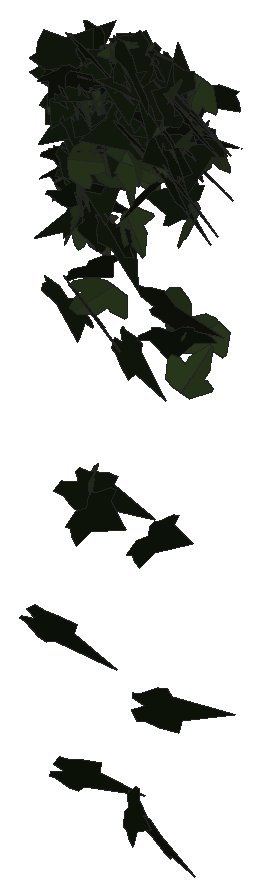
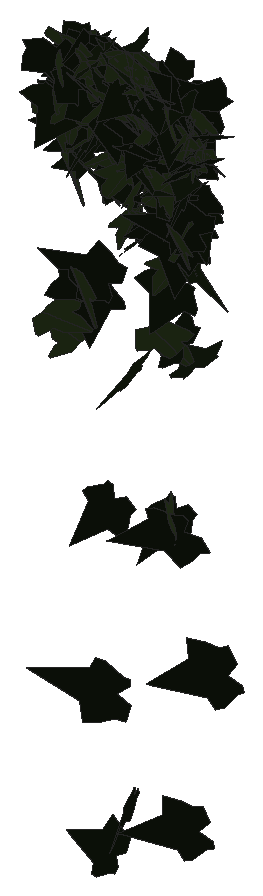
# SketchUp Ruby script. Lengths in inches.
U = 1.inch
M = Sketchup.active_model
def pt(a) = Geom::Point3d.new(a.map { |v| v * U })
def face(e, loops, mat)
  f = e.add_face(loops[0].map { |a| pt(a) })
  loops[1..].each { |l| e.add_face(l.map { |a| pt(a) }).erase! }
  f.material = f.back_material = mat if mat
  f
end
# faces: each face lists its corners as indices into pts; further lists are holes
def faces(e, pts, list, mat = nil) = list.each { |f| face(e, (f[0].is_a?(Array) ? f : [f]).map { |l| l.map { |i| pts[i] } }, mat) }
# xy, xz, yz: faces in a plane at the given z, y or x. An outline is a flat list of corners, or four numbers for a rectangle; further outlines are holes
def ring(l) = l.size == 4 ? [[l[0], l[1]], [l[2], l[1]], [l[2], l[3]], [l[0], l[3]]] : l.each_slice(2).to_a
def flat(e, list, mat, &to3) = list.each { |f| face(e, (f[0].is_a?(Array) ? f : [f]).map { |l| ring(l).map { |u, v| to3.(u, v) } }, mat) }
def xy(e, z, list, mat = nil) = flat(e, list, mat) { |x, y| [x, y, z] }
def xz(e, y, list, mat = nil) = flat(e, list, mat) { |x, z| [x, y, z] }
def yz(e, x, list, mat = nil) = flat(e, list, mat) { |y, z| [x, y, z] }
def lines(e, pts, list) = list.each { |a, b| e.add_line(pt(pts[a]), pt(pts[b])) }
# prism: a flat outline (further loops are holes) pulled along v
def prism(e, loops, v, mat = nil)
  f = face(e, loops, mat); d = Geom::Vector3d.new(v.map { |x| x * U })
  f.pushpull(f.normal.samedirection?(d) ? d.length : -d.length)
end
def box(e, o, s, mat = nil) = prism(e, [[o, [o[0] + s[0], o[1], o[2]], [o[0] + s[0], o[1] + s[1], o[2]], [o[0], o[1] + s[1], o[2]]]], [0, 0, s[2]], mat)
def at(x, y, z, deg = 0) = Geom::Transformation.translation(pt([x, y, z])) * Geom::Transformation.rotation(ORIGIN, Z_AXIS, deg.degrees)
def axes(o, x, y, z) = Geom::Transformation.new([*x, 0, *y, 0, *z, 0, *pt(o).to_a, 1])
def part(name) = M.definitions.add(name)
# library, detail: a bought-in or finely detailed component or shape, given as its bounding box
def library(name, o, s) = part(name).tap { |d| box(d.entities, o, s) }
def detail(e, o, s) = box(e.add_group.entities, o, s)
def put(e, d, t, mat = nil) = e.add_instance(d, t).tap { |i| i.material = mat if mat }
def group(e, t, mat = nil) = e.add_group.tap { |g| g.transformation = t; g.material = mat if mat }.entities
root = M.entities
M.materials.add("1026 AP 7946 SUNNY SIDE UP").color = [254, 231, 186]
M.materials.add("efeu1").color = [18, 25, 13]
M.materials.add("efeu2").color = [43, 57, 29]
c1 = part("ivyleaf_9")
p = [[1.54,2.16,1.25],[1.36,2.04,1.19],[-0.21,0.99,0.68],[-0.71,1.11,0.82],[-0.85,0.86,0.67],[-0.8,0.17,0.21],
  [-0.9,-0.01,0.1],[-0.67,-0.16,-0.02],[-0.08,-0.08,-0.05],[-0.03,-0.6,-0.4],[0.65,-0.88,-0.66],[0.83,-0.6,-0.49],
  [1.29,-0.42,-0.43],[1.8125,-0.07,-0.26],[1.21,0.44,0.15]]
faces(c1.entities,p,[[0,1,2,3,4,5,6,7,8,9,10,11,12,13,14]],"efeu1")
c2 = part("ivyleaf_10")
p = [[0,0.5,-0.03],[-0.0625,2.02,-0.43],[-0.19,2.01,-0.46],[-0.54,1.05,-0.29],[-0.52,0.625,-0.18],[-0.83,0.76,-0.28],
  [-1.16,0.64,-0.33],[-1.15,0.33,-0.24],[-0.77,-0.39,0.02],[-0.3,-0.51,0.16],[0.04,-0.48,0.23],[-0.02,2.01,-0.4375],
  [-0.06,2.01,-0.43],[0.04,-0.49,0.23],[0.67,-0.49,0.14],[1.38,0.36,-0.2],[1.375,0.51,-0.24],[0.81,0.65,-0.19],
  [0.62,0.59,-0.15],[0.6,1.09,-0.28],[0.5,1.23,-0.31]]
faces(c2.entities,p,[[0,1,2,3,4,5,6,7,8,9,10],[11,12,0,13,14,15,16,17,18,19,20]],"efeu2")
put(root,c1,axes([115.99,212.79,265.13],[-0.26427,0.17378,-0.05121],[0.02717,-0.05346,-0.24811],[-0.28334,-0.16721,0.02397]),"1026 AP 7946 SUNNY SIDE UP")
put(root,c1,axes([115.74,212.99,266.61],[-0.0821,-0.23949,0.03265],[-0.00331,-0.03337,-0.25266],[0.38014,-0.05201,0.00485]),"1026 AP 7946 SUNNY SIDE UP")
put(root,c2,axes([115.73,212.88,266.77],[0.19919,0.21849,0.01482],[0.02802,0.00485,-0.25981],[-0.34304,0.12727,-0.01262]),"1026 AP 7946 SUNNY SIDE UP")
put(root,c1,axes([115.8125,212.93,267.01],[-0.23551,-0.2009,0.04173],[0.02399,-0.06233,-0.25357],[0.32172,-0.14242,0.04946]),"1026 AP 7946 SUNNY SIDE UP")
put(root,c1,axes([115.93,212.68,265.9],[0.01878,0.24384,-0.04183],[-0.01659,-0.0415,-0.2516],[-0.38871,0.01355,0.00872]),"1026 AP 7946 SUNNY SIDE UP")
put(root,c2,axes([115.85,212.9,265.35],[0.05116,0.23767,-0.06271],[0.01151,0.0618,0.24749],[0.38613,-0.03333,0.00093]),"1026 AP 7946 SUNNY SIDE UP")
put(root,c1,axes([115.81,212.93,266.33],[0.24825,-0.13578,-0.18185],[-0.24069,0.08971,-0.21253],[0.25302,0.21856,-0.02375]),"1026 AP 7946 SUNNY SIDE UP")
put(root,c1,axes([115.68,212.91,263.6875],[-0.0167,-0.20611,0.14387],[0.09275,-0.13903,-0.20586],[0.38139,0.02479,0.05636]),"1026 AP 7946 SUNNY SIDE UP")
put(root,c1,axes([115.52,212.53,258.98],[0.41358,-0.02859,0.1247],[0.18193,-0.04871,-0.27076],[0.07246,0.28548,-0.03197]),"1026 AP 7946 SUNNY SIDE UP")
put(root,c2,axes([115.88,213.13,265.69],[0.27606,-0.17043,-0.00359],[-0.02245,-0.01111,-0.25146],[0.26707,0.17523,-0.01743]),"1026 AP 7946 SUNNY SIDE UP")
put(root,c2,axes([115.83,212.89,267.06],[-0.03773,0.24961,-0.05464],[0.00008,-0.05469,-0.2586],[-0.40172,-0.02346,0.00508]),"1026 AP 7946 SUNNY SIDE UP")
put(root,c1,axes([115.65,213,266.52],[0.28935,-0.16498,-0.02634],[0.01885,0.04965,-0.25011],[0.26162,0.17889,0.04715]),"1026 AP 7946 SUNNY SIDE UP")
put(root,c2,axes([115.875,212.79,267.35],[0.37173,-0.10682,0.00444],[-0.00745,-0.02238,-0.26639],[0.16798,0.2354,-0.02164]),"1026 AP 7946 SUNNY SIDE UP")
put(root,c2,axes([115.79,212.91,266.5625],[-0.13441,0.1576,-0.18274],[0.10829,-0.16494,-0.18519],[-0.35814,-0.10902,0.01259]),"1026 AP 7946 SUNNY SIDE UP")
put(root,c1,axes([115.74,212.92,266.82],[0.10246,-0.24103,0.0478],[-0.00107,-0.04959,-0.25714],[0.38636,0.06378,-0.01339]),"1026 AP 7946 SUNNY SIDE UP")
put(root,c1,axes([115.64,212.97,265.6875],[0.15087,0.01394,0.23225],[0.35005,0.03508,-0.09967],[-0.05933,0.24241,0.00252]),"1026 AP 7946 SUNNY SIDE UP")
put(root,c2,axes([116.03,212.91,267.03],[0.28883,-0.12781,-0.12018],[-0.14742,0.06823,-0.23013],[0.22779,0.20622,0.00345]),"1026 AP 7946 SUNNY SIDE UP")
put(root,c1,axes([115.96,212.9,265.45],[0.15048,0.22625,-0.03636],[-0.00526,-0.03826,-0.25301],[-0.36034,0.09504,-0.01149]),"1026 AP 7946 SUNNY SIDE UP")
put(root,c1,axes([116.01,212.66,266.07],[0.25903,0.14712,-0.11483],[-0.12722,-0.07798,-0.22796],[-0.26175,0.18349,-0.00284]),"1026 AP 7946 SUNNY SIDE UP")
put(root,c1,axes([115.75,212.83,266.95],[0.19134,-0.21265,0.06418],[0.04405,-0.05713,-0.2527],[0.34617,0.12481,-0.00332]),"1026 AP 7946 SUNNY SIDE UP")
put(root,c1,axes([115.83,212.66,267.36],[-0.1452,-0.01813,0.27512],[0.39855,0.08523,0.09671],[-0.13579,0.26952,-0.01033]),"1026 AP 7946 SUNNY SIDE UP")
put(root,c1,axes([115.84,212.97,266.64],[-0.1131,-0.19479,-0.14542],[0.14339,0.11304,-0.20955],[0.34892,-0.10959,0.03898]),"1026 AP 7946 SUNNY SIDE UP")
put(root,c1,axes([116.11,212.56,267.42],[0.03387,0.22555,-0.15246],[-0.01506,-0.14902,-0.23425],[-0.42503,0.02325,-0.00385]),"1026 AP 7946 SUNNY SIDE UP")
put(root,c2,axes([115.97,212.67,265.74],[-0.22116,0.20193,-0.02831],[0.00589,-0.03221,-0.25322],[-0.32063,-0.13987,0.01488]),"1026 AP 7946 SUNNY SIDE UP")
put(root,c2,axes([116.05,212.9,266.75],[-0.38906,-0.02119,0.00829],[-0.00969,-0.0233,-0.2549],[0.03437,-0.24646,0.02192]),"1026 AP 7946 SUNNY SIDE UP")
put(root,c2,axes([115.85,212.77,267.05],[0.24228,-0.14413,0.1453],[0.20469,-0.0658,-0.21491],[0.24335,0.19884,0.0361]),"1026 AP 7946 SUNNY SIDE UP")
put(root,c1,axes([115.91,212.76,266.07],[0.14209,-0.18673,-0.17045],[-0.12451,0.14422,-0.21275],[0.37084,0.11997,-0.00612]),"1026 AP 7946 SUNNY SIDE UP")
put(root,c1,axes([115.97,212.8,267.56],[0.3184,-0.03652,-0.16831],[-0.21748,0.10742,-0.20096],[0.14774,0.23683,0.0669]),"1026 AP 7946 SUNNY SIDE UP")
put(root,c2,axes([115.91,212.82,267.04],[-0.16774,0.12497,-0.19879],[0.14491,-0.17248,-0.16796],[-0.33219,-0.13834,0.02711]),"1026 AP 7946 SUNNY SIDE UP")
put(root,c1,axes([116.12,212.88,267.32],[0.11497,0.24742,0.00913],[-0.02443,0.01234,-0.26504],[-0.38846,0.07245,0.01937]),"1026 AP 7946 SUNNY SIDE UP")
put(root,c2,axes([116.07,212.93,267.26],[0.1152,-0.24189,0.03713],[0.00491,-0.03812,-0.26046],[0.38484,0.07289,-0.00779]),"1026 AP 7946 SUNNY SIDE UP")
put(root,c1,axes([115.77,212.8,256.69],[0.30915,0.03578,0.17193],[0.2621,0.01308,-0.20536],[-0.05629,0.25743,-0.01193]),"1026 AP 7946 SUNNY SIDE UP")
put(root,c1,axes([116.01,212.51,267.3],[0.34993,0.11273,-0.05787],[-0.06457,-0.04424,-0.2564],[-0.1877,0.22538,-0.01968]),"1026 AP 7946 SUNNY SIDE UP")
put(root,c1,axes([116.27,212.69,266.81],[-0.3998,0.01461,-0.01354],[0.01831,-0.02673,-0.26116],[-0.025,-0.2532,0.02528]),"1026 AP 7946 SUNNY SIDE UP")
put(root,c2,axes([116.11,212.62,265.28],[0.16821,-0.23293,0.01392],[-0.00471,-0.01769,-0.26396],[0.36697,0.10654,-0.00977]),"1026 AP 7946 SUNNY SIDE UP")
put(root,c2,axes([116.26,212.96,263.98],[0.28372,0.08808,-0.15619],[-0.24366,-0.02318,-0.20333],[-0.13046,0.23485,0.04009]),"1026 AP 7946 SUNNY SIDE UP")
put(root,c1,axes([116.35,212.82,267.75],[0.08478,-0.02272,-0.2649],[-0.40567,-0.00243,-0.05555],[0.00357,0.26259,-0.02189]),"1026 AP 7946 SUNNY SIDE UP")
put(root,c1,axes([115.98,212.99,266.35],[0.13622,-0.22035,-0.07713],[-0.00402,0.07766,-0.24211],[0.36527,0.08303,0.02609]),"1026 AP 7946 SUNNY SIDE UP")
put(root,c1,axes([116.46,213.05,266.52],[-0.06685,0.10519,0.22873],[-0.35852,0.06559,-0.07682],[-0.1416,-0.21573,0.0865]),"1026 AP 7946 SUNNY SIDE UP")
put(root,c2,axes([115.98,212.9,265.48],[-0.1779,-0.07484,0.21402],[0.241,0.14209,0.13927],[-0.25083,0.1896,-0.01799]),"1026 AP 7946 SUNNY SIDE UP")
put(root,c2,axes([116.1,212.79,265.01],[0.10908,0.20772,0.12034],[0.03741,0.11378,-0.22461],[-0.37194,0.07236,0.0127]),"1026 AP 7946 SUNNY SIDE UP")
put(root,c2,axes([116.17,212.6875,265.82],[0.00457,0.24817,0.00995],[-0.0331,0.00846,-0.2547],[-0.38903,0.0022,0.02179]),"1026 AP 7946 SUNNY SIDE UP")
put(root,c1,axes([115.95,212.55,265.5625],[0.33248,0.06838,0.14298],[0.2139,0.02844,-0.2284],[-0.11476,0.25111,-0.01147]),"1026 AP 7946 SUNNY SIDE UP")
put(root,c2,axes([116.11,213.09,266.27],[-0.2836,0.1109,-0.13053],[0.13323,-0.10173,-0.2155],[-0.22967,-0.19595,0.03618]),"1026 AP 7946 SUNNY SIDE UP")
put(root,c1,axes([115.99,212.93,267.02],[0.21513,-0.20751,0.05555],[0.0438,-0.04763,-0.25632],[0.33474,0.13959,-0.00216]),"1026 AP 7946 SUNNY SIDE UP")
put(root,c1,axes([116.09,212.78,265.95],[0.04147,0.24823,-0.01367],[-0.00152,0.01486,0.25724],[0.391,-0.02627,0.00245]),"1026 AP 7946 SUNNY SIDE UP")
put(root,c1,axes([116.04,212.73,266.59],[0.20331,-0.19533,-0.12397],[-0.02127,0.13018,-0.23406],[0.3592,0.11827,0.05631]),"1026 AP 7946 SUNNY SIDE UP")
put(root,c2,axes([116.12,212.85,261.11],[0.02743,-0.07559,-0.24836],[0.09658,-0.23269,0.07853],[-0.38469,-0.06381,0.002]),"1026 AP 7946 SUNNY SIDE UP")
put(root,c2,axes([116.08,212.84,267.21],[-0.12974,0.01526,-0.24756],[0.17464,-0.22307,-0.05516],[-0.33609,-0.1218,0.0669]),"1026 AP 7946 SUNNY SIDE UP")
put(root,c1,axes([115.99,212.83,263.84],[0.17739,-0.19459,0.15429],[0.10999,-0.13379,-0.23243],[0.37121,0.13263,-0.00486]),"1026 AP 7946 SUNNY SIDE UP")
put(root,c1,axes([115.99,212.83,261.07],[0.04321,0.01041,-0.2687],[0.2231,0.21962,0.02571],[0.34463,-0.14348,0.01705]),"1026 AP 7946 SUNNY SIDE UP")
put(root,c1,axes([116.46,212.94,267.23],[-0.27554,0.17764,-0.04819],[0.02815,-0.04921,-0.2564],[-0.28787,-0.17484,0.02105]),"1026 AP 7946 SUNNY SIDE UP")
put(root,c2,axes([116.3,212.87,267.03],[0.12383,-0.24045,0.02206],[0.00316,-0.02331,-0.26073],[0.37976,0.0786,-0.00502]),"1026 AP 7946 SUNNY SIDE UP")
put(root,c1,axes([116.28,212.6,264.53],[0.16063,0.21557,0.06768],[0.06015,0.05314,-0.24516],[-0.34864,0.10848,-0.01111]),"1026 AP 7946 SUNNY SIDE UP")
put(root,c1,axes([116.24,212.83,265.96],[-0.17523,-0.20346,-0.11103],[0.10768,0.08369,-0.23777],[0.34476,-0.12955,0.01783]),"1026 AP 7946 SUNNY SIDE UP")
put(root,c1,axes([116.53,212.87,267.34],[-0.38732,-0.032,0.05291],[-0.06927,-0.05383,-0.25165],[0.06559,-0.24584,0.04669]),"1026 AP 7946 SUNNY SIDE UP")
put(root,c1,axes([116.6,212.94,267.03],[-0.33606,0.12929,0.0196],[-0.0562,-0.02418,-0.2543],[-0.19748,-0.21314,0.03901]),"1026 AP 7946 SUNNY SIDE UP")
put(root,c2,axes([116.32,212.375,266.21],[0.01878,0.09821,0.27964],[-0.02414,0.27095,-0.09892],[-0.45243,-0.01038,0.01689]),"1026 AP 7946 SUNNY SIDE UP")
put(root,c1,axes([116.12,212.6875,267.65],[0.26987,-0.15445,0.11677],[0.11582,-0.08855,-0.23789],[0.27897,0.18618,-0.01419]),"1026 AP 7946 SUNNY SIDE UP")
put(root,c2,axes([116.36,212.9375,266.97],[0.03906,0.24632,-0.03327],[-0.01911,-0.03262,-0.25508],[-0.39046,0.02624,0.00915]),"1026 AP 7946 SUNNY SIDE UP")
put(root,c2,axes([116.14,212.79,265.94],[-0.04204,-0.04059,-0.25612],[0.36305,-0.10336,-0.00881],[-0.15748,-0.22743,0.04806]),"1026 AP 7946 SUNNY SIDE UP")
put(root,c1,axes([116.44,212.4,261.03],[0.00101,-0.03913,-0.2949],[-0.1883,0.26023,-0.03543],[0.41306,0.11873,-0.01543]),"1026 AP 7946 SUNNY SIDE UP")
put(root,c2,axes([116.54,212.8,266.97],[0.33305,0.06699,-0.11686],[-0.17262,-0.03025,-0.229],[-0.11542,0.23854,0.0053]),"1026 AP 7946 SUNNY SIDE UP")
put(root,c2,axes([116.375,212.94,267.18],[0.25069,0.19209,0.01986],[0.0344,0.00545,-0.25677],[-0.30143,0.16037,-0.01279]),"1026 AP 7946 SUNNY SIDE UP")
put(root,c1,axes([116.41,212.91,266.96],[0.29693,0.16118,-0.03177],[-0.01494,-0.03758,-0.25496],[-0.25788,0.18776,-0.02181]),"1026 AP 7946 SUNNY SIDE UP")
put(root,c1,axes([116.61,212.58,265],[0.19625,-0.0566,0.22905],[-0.21992,0.18231,0.12957],[-0.28658,-0.17866,0.05742]),"1026 AP 7946 SUNNY SIDE UP")
put(root,c2,axes([116.42,212.84,267.37],[-0.28461,-0.14573,-0.12344],[0.19749,0.02934,-0.23367],[0.22026,-0.21462,0.05002]),"1026 AP 7946 SUNNY SIDE UP")
put(root,c2,axes([116.5625,212.875,267.22],[0.02893,-0.25307,0.02157],[-0.0018,-0.02252,-0.26151],[0.39947,0.01823,-0.00274]),"1026 AP 7946 SUNNY SIDE UP")
put(root,c2,axes([116.52,212.97,267.23],[0.39386,0.0059,-0.0066],[-0.00919,-0.02411,-0.25708],[-0.01021,0.2494,-0.02322]),"1026 AP 7946 SUNNY SIDE UP")
put(root,c2,axes([116.52,212.93,267.25],[-0.35122,-0.09305,-0.06991],[0.12925,-0.02666,-0.24311],[0.12614,-0.23176,0.05444]),"1026 AP 7946 SUNNY SIDE UP")
put(root,c1,axes([116.55,213.03,266.39],[-0.17477,-0.20588,0.08334],[0.06975,-0.11062,-0.22463],[0.34144,-0.08279,0.08855]),"1026 AP 7946 SUNNY SIDE UP")
put(root,c2,axes([116.6875,212.92,267.46],[0.25476,-0.18856,-0.06594],[-0.07725,0.04069,-0.25565],[0.30288,0.16898,-0.00974]),"1026 AP 7946 SUNNY SIDE UP")
put(root,c2,axes([116.67,212.75,267.63],[-0.37006,0.11556,0.00982],[-0.02712,-0.01505,-0.26932],[-0.18021,-0.23504,0.02036]),"1026 AP 7946 SUNNY SIDE UP")
put(root,c2,axes([116.58,212.74,267.69],[-0.25114,0.17825,-0.09678],[0.06907,-0.0875,-0.24585],[-0.30996,-0.16392,0.02363]),"1026 AP 7946 SUNNY SIDE UP")
put(root,c2,axes([116.64,212.97,266.55],[0.26544,-0.18403,0.00743],[0.00824,-0.0064,-0.2573],[0.28954,0.16889,0.00051]),"1026 AP 7946 SUNNY SIDE UP")
put(root,c1,axes([116.66,212.67,266.58],[0.33243,0.06039,-0.12348],[-0.16669,-0.06306,-0.22508],[-0.13022,0.23488,-0.02711]),"1026 AP 7946 SUNNY SIDE UP")
put(root,c2,axes([116.71,212.95,267.3],[0.1599,-0.22636,0.04932],[0.01212,-0.05036,-0.25557],[0.36402,0.10111,-0.01316]),"1026 AP 7946 SUNNY SIDE UP")
put(root,c1,axes([116.91,212.95,267.77],[-0.36797,0.10412,-0.0168],[0.00796,-0.03,-0.26276],[-0.16568,-0.2327,0.0247]),"1026 AP 7946 SUNNY SIDE UP")
put(root,c2,axes([116.67,212.89,266.01],[-0.0718,0.24432,-0.03712],[0.00154,-0.03787,-0.2562],[-0.38864,-0.04528,0.00585]),"1026 AP 7946 SUNNY SIDE UP")
put(root,c1,axes([116.64,212.86,267.49],[0.26164,0.16367,0.10206],[0.0733,0.0914,-0.23793],[-0.29099,0.17019,0.03183]),"1026 AP 7946 SUNNY SIDE UP")
put(root,c2,axes([116.79,212.93,267.8],[-0.22796,-0.2095,0.04091],[0.02044,-0.05801,-0.25901],[0.33501,-0.13901,0.04364]),"1026 AP 7946 SUNNY SIDE UP")
put(root,c2,axes([116.91,212.7,266.46],[-0.31472,-0.10728,0.11538],[-0.13911,-0.07241,-0.23349],[0.20114,-0.21794,0.01905]),"1026 AP 7946 SUNNY SIDE UP")
put(root,c1,axes([116.63,212.93,263.33],[0.244,-0.18107,-0.13486],[-0.11464,0.1083,-0.24465],[0.3311,0.17094,0.01468]),"1026 AP 7946 SUNNY SIDE UP")
put(root,c2,axes([116.875,212.92,267.78],[-0.36609,-0.09921,0.05694],[-0.05982,-0.052,-0.25891],[0.16872,-0.23371,0.03175]),"1026 AP 7946 SUNNY SIDE UP")
put(root,c1,axes([116.67,212.78,267.625],[-0.20275,-0.1923,-0.11673],[0.20674,0.03889,-0.22406],[0.28253,-0.16645,0.08019]),"1026 AP 7946 SUNNY SIDE UP")
put(root,c1,axes([116.95,212.79,266.71],[-0.25785,-0.07647,0.18284],[-0.15383,-0.16848,-0.16848],[0.26278,-0.17366,0.08077]),"1026 AP 7946 SUNNY SIDE UP")
put(root,c1,axes([116.68,212.71,265.17],[0.07372,-0.24459,0.0058],[0.00399,-0.00666,-0.2566],[0.38473,0.04693,0.00155]),"1026 AP 7946 SUNNY SIDE UP")
put(root,c1,axes([117.03,212.79,267.86],[-0.38899,0.0636,-0.03909],[0.05099,-0.02733,-0.26263],[-0.10502,-0.24884,0.01729]),"1026 AP 7946 SUNNY SIDE UP")
put(root,c1,axes([116.81,212.98,267.4375],[-0.24959,-0.17248,-0.09984],[0.1319,0.05248,-0.23988],[0.28092,-0.17789,0.02393]),"1026 AP 7946 SUNNY SIDE UP")
put(root,c2,axes([116.88,212.65,266.49],[-0.36144,0.09559,-0.03084],[0.02846,-0.03543,-0.25531],[-0.15517,-0.22915,0.025]),"1026 AP 7946 SUNNY SIDE UP")
put(root,c2,axes([116.83,212.91,266.17],[0.11604,0.21625,0.11152],[0.0513,0.10195,-0.23479],[-0.37591,0.08066,0.00238]),"1026 AP 7946 SUNNY SIDE UP")
put(root,c1,axes([116.99,212.59,256.65],[0.12231,-0.05097,-0.24621],[-0.26718,0.16855,-0.09313],[0.27553,0.18607,0.01898]),"1026 AP 7946 SUNNY SIDE UP")
put(root,c2,axes([116.74,212.94,266.71],[0.27832,-0.02744,0.18002],[0.26293,-0.05531,-0.1836],[0.09143,0.24261,-0.01999]),"1026 AP 7946 SUNNY SIDE UP")
put(root,c2,axes([116.92,212.68,265.39],[0.01088,0.24279,0.0609],[-0.01137,0.05793,-0.24972],[-0.39224,0.00506,0.00893]),"1026 AP 7946 SUNNY SIDE UP")
put(root,c1,axes([117.22,212.94,266.94],[-0.33821,-0.0355,0.13007],[-0.18611,-0.05282,-0.22297],[0.08955,-0.24386,0.02784]),"1026 AP 7946 SUNNY SIDE UP")
put(root,c1,axes([117.19,212.91,267.47],[-0.18089,0.22509,0.0191],[-0.01993,0.01291,-0.26029],[-0.35442,-0.11561,0.00489]),"1026 AP 7946 SUNNY SIDE UP")
put(root,c1,axes([117.13,212.9,267.79],[-0.34043,0.06657,-0.11902],[0.12092,-0.11843,-0.21875],[-0.17191,-0.21513,0.08183]),"1026 AP 7946 SUNNY SIDE UP")
put(root,c1,axes([116.82,212.62,266.74],[0.36267,-0.09843,-0.01243],[-0.02796,-0.01242,-0.25772],[0.1533,0.2306,-0.01759]),"1026 AP 7946 SUNNY SIDE UP")
put(root,c1,axes([117.17,212.97,267.09],[0.12691,0.22233,-0.0891],[-0.11286,-0.0658,-0.24015],[-0.3585,0.09942,0.04406]),"1026 AP 7946 SUNNY SIDE UP")
put(root,c1,axes([116.88,212.76,267.79],[0.09352,-0.23225,0.11039],[0.01961,-0.1086,-0.24722],[0.40258,0.05924,-0.0136]),"1026 AP 7946 SUNNY SIDE UP")
put(root,c2,axes([117.15,212.99,267.67],[0.29264,0.13087,-0.11726],[-0.14401,-0.06891,-0.23476],[-0.2325,0.2074,-0.00218]),"1026 AP 7946 SUNNY SIDE UP")
put(root,c1,axes([117.22,212.77,265.98],[-0.16422,0.17191,-0.15567],[0.108,-0.13603,-0.20778],[-0.34437,-0.12464,0.00908]),"1026 AP 7946 SUNNY SIDE UP")
put(root,c1,axes([116.98,212.8,267.63],[0.02539,-0.25272,-0.00041],[0.05569,0.00124,-0.25831],[0.39346,0.01613,0.03659]),"1026 AP 7946 SUNNY SIDE UP")
put(root,c1,axes([117.52,212.84,267.17],[-0.07931,-0.05439,-0.30495],[-0.43858,-0.10348,0.06802],[-0.1765,0.28156,-0.03198]),"1026 AP 7946 SUNNY SIDE UP")
put(root,c2,axes([116.98,212.64,266.28],[-0.06298,-0.11169,-0.23114],[0.29646,0.13536,-0.10359],[0.2583,-0.18259,0.06254]),"1026 AP 7946 SUNNY SIDE UP")
put(root,c1,axes([116.89,213.11,256.09],[0.19949,-0.15186,0.18798],[0.1537,-0.15619,-0.20389],[0.34132,0.1591,-0.01805]),"1026 AP 7946 SUNNY SIDE UP")
put(root,c2,axes([117.17,212.98,267.02],[-0.02725,0.24806,0.04222],[0.0039,0.03983,-0.25588],[-0.39496,-0.01672,-0.00544]),"1026 AP 7946 SUNNY SIDE UP")
put(root,c2,axes([117.28,212.875,267.39],[-0.09412,-0.24062,0.07595],[-0.01842,-0.07444,-0.2558],[0.39593,-0.06066,0.00615]),"1026 AP 7946 SUNNY SIDE UP")
put(root,c1,axes([117.14,212.82,267.35],[-0.0099,-0.22172,0.12138],[-0.00452,-0.11904,-0.2292],[0.39571,-0.00691,0.00042]),"1026 AP 7946 SUNNY SIDE UP")
put(root,c1,axes([117.56,212.92,267.15],[-0.23937,0.15587,0.13832],[-0.17309,0.07809,-0.22299],[-0.2722,-0.18673,0.02016]),"1026 AP 7946 SUNNY SIDE UP")
put(root,c1,axes([117.3,212.7,267.47],[0.30769,0.16265,-0.0099],[0.0062,-0.02118,-0.26154],[-0.25621,0.19482,-0.01822]),"1026 AP 7946 SUNNY SIDE UP")
put(root,c1,axes([117.39,212.51,260.91],[-0.04033,0.02337,-0.28882],[-0.15471,0.26314,0.03339],[0.41465,0.10045,-0.01563]),"1026 AP 7946 SUNNY SIDE UP")
put(root,c1,axes([117.75,212.63,267.62],[-0.3017,0.05383,0.19025],[-0.29311,0.01058,-0.20298],[-0.07275,-0.26589,0.02882]),"1026 AP 7946 SUNNY SIDE UP")
put(root,c1,axes([117.51,212.64,267.12],[0.25675,0.12972,-0.14961],[-0.19528,-0.07785,-0.21485],[-0.23696,0.20471,0.01495]),"1026 AP 7946 SUNNY SIDE UP")
put(root,c1,axes([117.36,212.89,266.54],[0.16107,-0.16369,-0.17114],[0.1523,-0.13408,0.19796],[-0.33245,-0.14073,0.00777]),"1026 AP 7946 SUNNY SIDE UP")
put(root,c1,axes([117.25,212.99,267.76],[0.18962,-0.22488,0.00151],[0.01478,0.00193,-0.2627],[0.35333,0.12061,0.01018]),"1026 AP 7946 SUNNY SIDE UP")
put(root,c1,axes([117.59,212.97,267.34],[-0.04676,0.22244,-0.12066],[-0.01321,-0.12002,-0.23084],[-0.39601,-0.02226,0.02195]),"1026 AP 7946 SUNNY SIDE UP")
put(root,c2,axes([117.42,212.77,267.375],[0.39658,-0.02394,-0.00354],[-0.00891,-0.02497,-0.25983],[0.03695,0.251,-0.02469]),"1026 AP 7946 SUNNY SIDE UP")
put(root,c1,axes([117.41,212.875,266.59],[0.22791,-0.14075,-0.1599],[-0.1929,0.09479,-0.20709],[0.26593,0.18939,-0.01318]),"1026 AP 7946 SUNNY SIDE UP")
put(root,c1,axes([117.2,212.72,258.21],[0.2181,0.12443,-0.21575],[0.18358,0.17847,0.1893],[0.33728,-0.1776,0.03648]),"1026 AP 7946 SUNNY SIDE UP")
put(root,c2,axes([117.64,212.88,264.26],[0.23923,-0.19429,-0.12999],[-0.10803,0.10495,-0.25343],[0.34691,0.16667,0.01073]),"1026 AP 7946 SUNNY SIDE UP")
put(root,c2,axes([117.57,212.92,266.78],[-0.28498,-0.17301,-0.04157],[0.08797,-0.00231,-0.25486],[0.26476,-0.18545,0.03993]),"1026 AP 7946 SUNNY SIDE UP")
put(root,c1,axes([117.85,212.69,265.98],[-0.20472,0.18591,0.11777],[-0.11562,0.08666,-0.23311],[-0.32218,-0.14923,0.00882]),"1026 AP 7946 SUNNY SIDE UP")
put(root,c2,axes([117.69,212.84,267.57],[0.27696,-0.18536,-0.05083],[-0.0708,0.02369,-0.26276],[0.29275,0.18109,-0.01547]),"1026 AP 7946 SUNNY SIDE UP")
put(root,c1,axes([117.7,212.6,264.03],[0.19728,0.20656,-0.0882],[-0.06474,-0.07652,-0.24938],[-0.3463,0.13198,-0.00362]),"1026 AP 7946 SUNNY SIDE UP")
put(root,c2,axes([117.66,212.75,267.58],[0.10921,-0.19936,0.16316],[0.07473,-0.15232,-0.21834],[0.39445,0.08406,-0.00381]),"1026 AP 7946 SUNNY SIDE UP")
put(root,c2,axes([117.8125,213.23,263.85],[0.17646,0.10744,-0.21272],[-0.22968,-0.14684,-0.16089],[-0.28606,0.18418,-0.00204]),"1026 AP 7946 SUNNY SIDE UP")
put(root,c1,axes([117.36,212.7,264.25],[0.19048,-0.08166,0.2315],[0.28884,-0.13028,-0.15124],[0.24172,0.22002,-0.00171]),"1026 AP 7946 SUNNY SIDE UP")
put(root,c1,axes([117.55,212.75,266.12],[0.25665,-0.19282,0.02251],[0.00157,-0.02914,-0.25976],[0.30532,0.16223,-0.01759]),"1026 AP 7946 SUNNY SIDE UP")
put(root,c1,axes([117.85,212.65,267.35],[-0.19961,-0.15763,0.21873],[0.17851,0.18132,0.20879],[-0.37679,0.16941,-0.01696]),"1026 AP 7946 SUNNY SIDE UP")
put(root,c2,axes([117.91,212.94,266.83],[-0.44356,0.08583,0.08957],[-0.14335,-0.00409,-0.30229],[-0.12706,-0.29501,0.02837]),"1026 AP 7946 SUNNY SIDE UP")
put(root,c1,axes([117.65,212.87,266.64],[-0.04823,-0.14813,0.21107],[0.05634,-0.20768,-0.14976],[0.39461,0.01155,0.04717]),"1026 AP 7946 SUNNY SIDE UP")
put(root,c2,axes([117.82,212.96,267.49],[0.04393,-0.25092,0.03275],[0.00538,-0.03304,-0.26028],[0.39795,0.02814,-0.0001]),"1026 AP 7946 SUNNY SIDE UP")
put(root,c1,axes([117.55,212.78,267.48],[0.21536,-0.2009,0.07406],[0.12416,-0.03305,-0.24642],[0.31235,0.15166,0.04689]),"1026 AP 7946 SUNNY SIDE UP")
put(root,c1,axes([117.94,212.96,267.61],[0.16049,0.1537,-0.18111],[-0.13538,-0.1546,-0.1907],[-0.34242,0.13316,-0.00949]),"1026 AP 7946 SUNNY SIDE UP")
put(root,c1,axes([117.79,212.89,266.88],[0.34503,0.13039,-0.01819],[-0.06934,0.03908,-0.25633],[-0.1951,0.21671,0.05893]),"1026 AP 7946 SUNNY SIDE UP")
put(root,c1,axes([117.57,212.89,266.63],[0.28668,-0.14828,0.10112],[0.11351,-0.06808,-0.2424],[0.25635,0.19598,-0.00576]),"1026 AP 7946 SUNNY SIDE UP")
put(root,c2,axes([117.9,212.88,266.99],[-0.01074,-0.25529,0.0238],[0.00217,-0.0246,-0.26323],[0.40327,-0.00667,0.00205]),"1026 AP 7946 SUNNY SIDE UP")
put(root,c1,axes([117.64,212.6,267.45],[0.34752,-0.12852,0.02298],[0.0157,-0.02852,-0.26278],[0.2047,0.22037,-0.01886]),"1026 AP 7946 SUNNY SIDE UP")
put(root,c1,axes([117.66,212.64,266.34],[0.30925,-0.17362,0.01569],[-0.00084,-0.02504,-0.26969],[0.27419,0.19574,-0.01852]),"1026 AP 7946 SUNNY SIDE UP")
put(root,c2,axes([117.8,212.73,263.27],[0.15261,0.15862,-0.20209],[0.14768,0.1734,0.19244],[0.36935,-0.13487,0.00656]),"1026 AP 7946 SUNNY SIDE UP")
put(root,c2,axes([117.9,212.82,267.69],[0.38782,-0.08473,-0.02336],[-0.04527,-0.01578,-0.2676],[0.13007,0.24714,-0.02348]),"1026 AP 7946 SUNNY SIDE UP")
put(root,c2,axes([117.93,212.73,265.81],[0.18433,-0.23334,-0.00693],[-0.01802,0.00028,-0.26881],[0.36656,0.11735,-0.00973]),"1026 AP 7946 SUNNY SIDE UP")
put(root,c1,axes([117.87,212.88,266.9375],[-0.29884,-0.07703,-0.15883],[0.25441,-0.0025,-0.20478],[0.09158,-0.24443,0.05058]),"1026 AP 7946 SUNNY SIDE UP")
put(root,c1,axes([117.8,212.63,267.55],[0.33234,-0.14341,0.03087],[0.02717,-0.02927,-0.26288],[0.22904,0.21157,-0.01361]),"1026 AP 7946 SUNNY SIDE UP")
